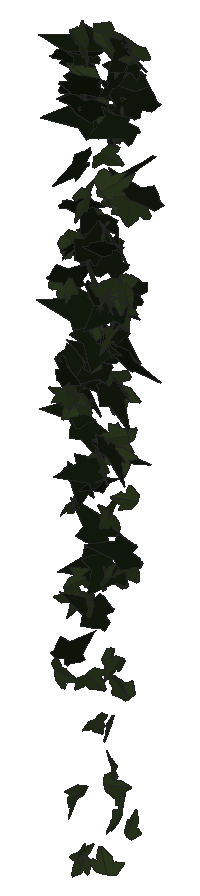
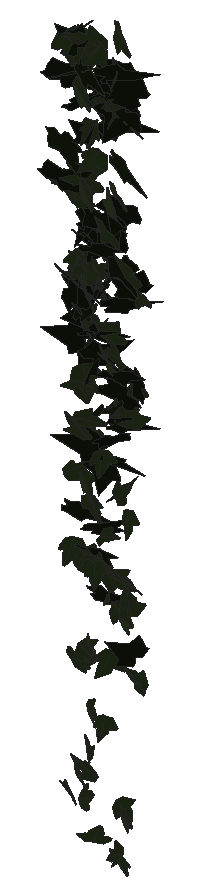
# SketchUp Ruby script. Lengths in inches.
U = 1.inch
M = Sketchup.active_model
def pt(a) = Geom::Point3d.new(a.map { |v| v * U })
def face(e, loops, mat)
  f = e.add_face(loops[0].map { |a| pt(a) })
  loops[1..].each { |l| e.add_face(l.map { |a| pt(a) }).erase! }
  f.material = f.back_material = mat if mat
  f
end
# faces: each face lists its corners as indices into pts; further lists are holes
def faces(e, pts, list, mat = nil) = list.each { |f| face(e, (f[0].is_a?(Array) ? f : [f]).map { |l| l.map { |i| pts[i] } }, mat) }
# xy, xz, yz: faces in a plane at the given z, y or x. An outline is a flat list of corners, or four numbers for a rectangle; further outlines are holes
def ring(l) = l.size == 4 ? [[l[0], l[1]], [l[2], l[1]], [l[2], l[3]], [l[0], l[3]]] : l.each_slice(2).to_a
def flat(e, list, mat, &to3) = list.each { |f| face(e, (f[0].is_a?(Array) ? f : [f]).map { |l| ring(l).map { |u, v| to3.(u, v) } }, mat) }
def xy(e, z, list, mat = nil) = flat(e, list, mat) { |x, y| [x, y, z] }
def xz(e, y, list, mat = nil) = flat(e, list, mat) { |x, z| [x, y, z] }
def yz(e, x, list, mat = nil) = flat(e, list, mat) { |y, z| [x, y, z] }
def lines(e, pts, list) = list.each { |a, b| e.add_line(pt(pts[a]), pt(pts[b])) }
# prism: a flat outline (further loops are holes) pulled along v
def prism(e, loops, v, mat = nil)
  f = face(e, loops, mat); d = Geom::Vector3d.new(v.map { |x| x * U })
  f.pushpull(f.normal.samedirection?(d) ? d.length : -d.length)
end
def box(e, o, s, mat = nil) = prism(e, [[o, [o[0] + s[0], o[1], o[2]], [o[0] + s[0], o[1] + s[1], o[2]], [o[0], o[1] + s[1], o[2]]]], [0, 0, s[2]], mat)
def at(x, y, z, deg = 0) = Geom::Transformation.translation(pt([x, y, z])) * Geom::Transformation.rotation(ORIGIN, Z_AXIS, deg.degrees)
def axes(o, x, y, z) = Geom::Transformation.new([*x, 0, *y, 0, *z, 0, *pt(o).to_a, 1])
def part(name) = M.definitions.add(name)
# library, detail: a bought-in or finely detailed component or shape, given as its bounding box
def library(name, o, s) = part(name).tap { |d| box(d.entities, o, s) }
def detail(e, o, s) = box(e.add_group.entities, o, s)
def put(e, d, t, mat = nil) = e.add_instance(d, t).tap { |i| i.material = mat if mat }
def group(e, t, mat = nil) = e.add_group.tap { |g| g.transformation = t; g.material = mat if mat }.entities
root = M.entities
M.materials.add("1026 AP 7946 SUNNY SIDE UP").color = [254, 231, 186]
M.materials.add("efeu1").color = [18, 25, 13]
M.materials.add("efeu2").color = [43, 57, 29]
c1 = part("ivyleaf_9")
p = [[1.54,2.16,1.25],[1.36,2.04,1.19],[-0.21,0.99,0.68],[-0.71,1.11,0.82],[-0.85,0.86,0.67],[-0.8,0.17,0.21],
  [-0.9,-0.01,0.1],[-0.67,-0.16,-0.02],[-0.08,-0.08,-0.05],[-0.03,-0.6,-0.4],[0.65,-0.88,-0.66],[0.83,-0.6,-0.49],
  [1.29,-0.42,-0.43],[1.8125,-0.07,-0.26],[1.21,0.44,0.15]]
faces(c1.entities,p,[[0,1,2,3,4,5,6,7,8,9,10,11,12,13,14]],"efeu1")
c2 = part("ivyleaf_10")
p = [[0,0.5,-0.03],[-0.0625,2.02,-0.43],[-0.19,2.01,-0.46],[-0.54,1.05,-0.29],[-0.52,0.625,-0.18],[-0.83,0.76,-0.28],
  [-1.16,0.64,-0.33],[-1.15,0.33,-0.24],[-0.77,-0.39,0.02],[-0.3,-0.51,0.16],[0.04,-0.48,0.23],[-0.02,2.01,-0.4375],
  [-0.06,2.01,-0.43],[0.04,-0.49,0.23],[0.67,-0.49,0.14],[1.38,0.36,-0.2],[1.375,0.51,-0.24],[0.81,0.65,-0.19],
  [0.62,0.59,-0.15],[0.6,1.09,-0.28],[0.5,1.23,-0.31]]
faces(c2.entities,p,[[0,1,2,3,4,5,6,7,8,9,10],[11,12,0,13,14,15,16,17,18,19,20]],"efeu2")
put(root,c1,axes([99.77,211.71,258.34],[0.11421,-0.24829,0.05884],[0.0227,-0.05675,-0.26683],[0.40047,0.07403,-0.00166]),"1026 AP 7946 SUNNY SIDE UP")
put(root,c1,axes([100.13,211.37,266.9],[0.01347,0.18196,0.23209],[-0.01628,0.21455,-0.19155],[-0.4771,-0.00219,0.01309]),"1026 AP 7946 SUNNY SIDE UP")
put(root,c1,axes([99.22,211.72,261.21],[-0.20633,0.02031,0.24724],[-0.36489,-0.10681,-0.11268],[0.14623,-0.23786,0.0677]),"1026 AP 7946 SUNNY SIDE UP")
put(root,c2,axes([98.75,211.59,259.34],[-0.065,-0.22355,-0.07009],[0.09307,0.0529,-0.23757],[0.38291,-0.0508,0.04585]),"1026 AP 7946 SUNNY SIDE UP")
put(root,c2,axes([99.16,211.6875,263.875],[0.2789,-0.19863,0.04906],[0.03014,-0.04802,-0.27606],[0.34574,0.16441,-0.01551]),"1026 AP 7946 SUNNY SIDE UP")
put(root,c2,axes([98.63,211.68,261.73],[0.34742,-0.07327,0.07071],[0.09567,-0.04065,-0.23245],[0.13876,0.21148,-0.01677]),"1026 AP 7946 SUNNY SIDE UP")
put(root,c1,axes([98.97,211.53,266.52],[0.37924,0.04384,0.16248],[0.25973,0.0013,-0.24242],[-0.06289,0.26976,-0.02137]),"1026 AP 7946 SUNNY SIDE UP")
put(root,c1,axes([100.32,211.7,256.1],[-0.11456,-0.07824,-0.20637],[-0.2718,-0.10819,0.10608],[-0.22297,0.17209,-0.02328]),"1026 AP 7946 SUNNY SIDE UP")
put(root,c2,axes([99.25,211.52,267.53],[-0.03367,0.04237,0.29564],[-0.39103,0.15321,-0.04082],[-0.26673,-0.22995,0.02253]),"1026 AP 7946 SUNNY SIDE UP")
put(root,c1,axes([99.125,211.71,264.66],[-0.32423,0.16869,-0.09489],[0.08807,-0.07794,-0.27385],[-0.28986,-0.21238,0.02294]),"1026 AP 7946 SUNNY SIDE UP")
put(root,c1,axes([99.38,211.76,257.61],[-0.32792,0.00418,0.0938],[-0.14856,-0.02146,-0.2059],[0.00862,-0.211,0.01982]),"1026 AP 7946 SUNNY SIDE UP")
put(root,c1,axes([99.86,211.79,261.62],[-0.42831,0.01177,-0.06642],[0.10133,-0.04083,-0.26808],[-0.03576,-0.25664,0.03592]),"1026 AP 7946 SUNNY SIDE UP")
put(root,c2,axes([99.64,211.7,261.84],[0.19511,-0.23098,-0.06612],[-0.05478,0.04954,-0.27543],[0.40086,0.1192,-0.00546]),"1026 AP 7946 SUNNY SIDE UP")
put(root,c1,axes([99.79,211.74,259.66],[0.10997,-0.2454,-0.0855],[-0.05012,0.07571,-0.26226],[0.40355,0.07628,-0.00927]),"1026 AP 7946 SUNNY SIDE UP")
put(root,c1,axes([100.0625,211.9,265.8],[-0.25059,-0.12748,0.18092],[-0.19412,-0.12774,-0.20985],[0.30507,-0.186,0.01508]),"1026 AP 7946 SUNNY SIDE UP")
put(root,c1,axes([98.43,211.8125,259.61],[0.17456,-0.11982,-0.18823],[0.345,0.00242,0.12665],[-0.09925,-0.20232,0.10918]),"1026 AP 7946 SUNNY SIDE UP")
put(root,c2,axes([99.34,211.62,262.38],[-0.24271,0.20597,0.10136],[-0.10582,0.0686,-0.2672],[-0.36803,-0.15556,0.00998]),"1026 AP 7946 SUNNY SIDE UP")
put(root,c1,axes([100.12,211.94,267.34],[-0.15431,-0.13846,0.2225],[-0.09689,-0.20573,-0.17483],[0.41533,-0.09944,0.04189]),"1026 AP 7946 SUNNY SIDE UP")
put(root,c2,axes([99.52,211.73,257.96],[-0.22827,0.18235,-0.06401],[0.03856,-0.06028,-0.24273],[-0.32477,-0.13533,0.01617]),"1026 AP 7946 SUNNY SIDE UP")
put(root,c1,axes([99.35,211.61,262.63],[-0.1499,-0.10114,0.24471],[0.27681,0.16226,0.14574],[-0.32428,0.18526,0.01129]),"1026 AP 7946 SUNNY SIDE UP")
put(root,c1,axes([99.39,211.58,262.86],[0.3039,0.19276,0.03365],[0.05358,0.01008,-0.28096],[-0.32651,0.18106,-0.01478]),"1026 AP 7946 SUNNY SIDE UP")
put(root,c2,axes([100.1875,211.84,267.28],[-0.08385,-0.22778,0.11653],[0.005,-0.11442,-0.24974],[0.43071,-0.04302,0.02559]),"1026 AP 7946 SUNNY SIDE UP")
put(root,c1,axes([99.19,211.68,266.08],[0.32051,0.12859,-0.14839],[-0.17988,-0.0931,-0.24535],[-0.26834,0.21601,-0.01277]),"1026 AP 7946 SUNNY SIDE UP")
put(root,c2,axes([99.29,211.67,252.9],[-0.16828,-0.16709,-0.1533],[0.13921,0.11873,-0.20354],[0.32203,-0.13864,0.00787]),"1026 AP 7946 SUNNY SIDE UP")
put(root,c2,axes([98.36,211.82,252.61],[-0.0983,0.03746,0.22474],[0.33412,-0.05251,0.07178],[0.09625,0.22056,-0.01968]),"1026 AP 7946 SUNNY SIDE UP")
put(root,c1,axes([98.63,211.68,261.77],[-0.03622,-0.04414,0.23863],[0.36392,0.07199,0.03814],[-0.13072,0.21263,0.04007]),"1026 AP 7946 SUNNY SIDE UP")
put(root,c2,axes([99.74,211.93,260.85],[0.03742,-0.16086,0.19473],[0.04663,-0.18193,-0.17635],[0.41223,0.03518,0.00227]),"1026 AP 7946 SUNNY SIDE UP")
put(root,c2,axes([99.85,211.84,262],[0.34797,-0.05261,0.13038],[0.19153,-0.05115,-0.2264],[0.12048,0.23324,-0.01666]),"1026 AP 7946 SUNNY SIDE UP")
put(root,c2,axes([99.74,211.77,261.83],[-0.28133,-0.16316,0.06208],[0.05116,0.05488,0.24908],[-0.26918,0.18096,-0.01754]),"1026 AP 7946 SUNNY SIDE UP")
put(root,c1,axes([99.54,211.8,254.375],[-0.24628,-0.09398,-0.16308],[-0.22319,-0.0696,0.18748],[-0.18319,0.21113,-0.00917]),"1026 AP 7946 SUNNY SIDE UP")
put(root,c2,axes([99.83,211.79,261.64],[-0.41731,0.03049,-0.08758],[0.12806,-0.05111,-0.26255],[-0.07583,-0.25412,0.03855]),"1026 AP 7946 SUNNY SIDE UP")
put(root,c1,axes([99.74,211.73,263.22],[0.3409,-0.08165,-0.15278],[-0.22589,0.04871,-0.23136],[0.16125,0.24087,-0.00112]),"1026 AP 7946 SUNNY SIDE UP")
put(root,c1,axes([99.16,211.98,265.65],[-0.06601,-0.11605,-0.26027],[-0.12972,-0.2381,0.12574],[-0.41648,0.09256,0.00209]),"1026 AP 7946 SUNNY SIDE UP")
put(root,c1,axes([99.39,211.96,260.625],[-0.26858,-0.19279,-0.01191],[0.06955,-0.02268,-0.26273],[0.32013,-0.15682,0.04709]),"1026 AP 7946 SUNNY SIDE UP")
put(root,c1,axes([100.39,211.9,266.26],[0.07581,0.0398,0.27726],[-0.43327,-0.05047,0.05483],[0.09667,-0.25739,0.02831]),"1026 AP 7946 SUNNY SIDE UP")
put(root,c1,axes([99.45,211.88,260.0625],[-0.39129,0.04731,-0.05286],[0.0733,-0.03669,-0.25081],[-0.091,-0.23299,0.02529]),"1026 AP 7946 SUNNY SIDE UP")
put(root,c2,axes([99.22,211.89,254.39],[-0.12233,0.18567,0.13228],[0.09489,-0.11261,0.20646],[0.34106,0.09792,-0.01]),"1026 AP 7946 SUNNY SIDE UP")
put(root,c1,axes([99.75,211.6875,262.41],[-0.34926,0.14547,0.01992],[0.04084,0.00516,0.26914],[0.24518,0.20636,-0.01645]),"1026 AP 7946 SUNNY SIDE UP")
put(root,c1,axes([99.43,211.7,257.375],[0.12713,0.19847,0.0268],[0.02228,0.01903,-0.22676],[-0.33832,0.07583,-0.00486]),"1026 AP 7946 SUNNY SIDE UP")
put(root,c1,axes([98.92,211.73,263.65],[0.24636,0.16085,-0.02269],[-0.00791,-0.02709,-0.23178],[-0.27578,0.14447,-0.01362]),"1026 AP 7946 SUNNY SIDE UP")
put(root,c2,axes([99.63,211.79,248.55],[0.25189,0.12326,0.02247],[-0.04422,0.00208,0.20735],[0.1916,-0.16157,0.01831]),"1026 AP 7946 SUNNY SIDE UP")
put(root,c2,axes([99.04,211.94,254.99],[-0.12494,-0.09685,0.18318],[-0.14224,-0.15456,-0.12888],[0.28568,-0.11932,0.01594]),"1026 AP 7946 SUNNY SIDE UP")
put(root,c2,axes([100.11,211.75,262.16],[-0.02207,0.25905,0.06742],[-0.04394,0.05815,-0.27584],[-0.44909,-0.01842,0.02367]),"1026 AP 7946 SUNNY SIDE UP")
put(root,c1,axes([99.65,211.95,255.4375],[-0.34728,-0.09961,-0.02051],[0.04243,-0.013,-0.24856],[0.1538,-0.22132,0.02227]),"1026 AP 7946 SUNNY SIDE UP")
put(root,c1,axes([99.26,211.85,261.77],[0.22541,-0.19793,-0.07928],[-0.0854,0.0522,-0.25411],[0.34687,0.14147,-0.01104]),"1026 AP 7946 SUNNY SIDE UP")
put(root,c1,axes([98.67,211.69,253.14],[-0.0515,-0.01577,0.25538],[0.3206,0.14127,0.03782],[-0.22334,0.20643,-0.00459]),"1026 AP 7946 SUNNY SIDE UP")
put(root,c2,axes([99.77,211.99,266.36],[-0.07588,0.07804,-0.24106],[0.12927,-0.21349,-0.09795],[-0.38505,-0.08705,0.01462]),"1026 AP 7946 SUNNY SIDE UP")
put(root,c2,axes([99.64,211.81,261.62],[-0.21057,0.22314,0.01514],[-0.03009,0.00298,-0.27286],[-0.37807,-0.12452,0.01328]),"1026 AP 7946 SUNNY SIDE UP")
put(root,c1,axes([98.75,212.04,257.13],[-0.02487,-0.2191,0.1306],[0.00606,-0.12846,-0.22676],[0.39897,-0.01171,0.01159]),"1026 AP 7946 SUNNY SIDE UP")
put(root,c2,axes([100.125,211.98,257.11],[0.01722,0.07495,0.19357],[-0.0502,-0.1774,0.07846],[0.32689,-0.03119,0.00185]),"1026 AP 7946 SUNNY SIDE UP")
put(root,c2,axes([100.2,211.87,263.98],[-0.40818,-0.04919,0.04791],[-0.06751,-0.03116,-0.26212],[0.0914,-0.24271,0.02035]),"1026 AP 7946 SUNNY SIDE UP")
put(root,c2,axes([99.86,211.85,258.14],[0.20478,0.16132,0.03611],[0.04892,0.01787,-0.21501],[-0.27474,0.12342,-0.01137]),"1026 AP 7946 SUNNY SIDE UP")
put(root,c2,axes([99.99,211.78,252.81],[-0.0923,0.04532,-0.19893],[-0.2138,0.13771,0.0771],[0.24563,0.13689,-0.00765]),"1026 AP 7946 SUNNY SIDE UP")
put(root,c2,axes([98.63,211.92,254.36],[-0.19793,-0.17291,-0.0116],[-0.0163,-0.00516,0.22023],[-0.27187,0.12619,-0.00476]),"1026 AP 7946 SUNNY SIDE UP")
put(root,c2,axes([99.83,212.01,258.47],[-0.05271,-0.02994,0.20973],[-0.15525,-0.17419,-0.04637],[0.29918,-0.09566,0.01289]),"1026 AP 7946 SUNNY SIDE UP")
put(root,c2,axes([98.94,211.91,248.4375],[0.26207,-0.11136,-0.03687],[-0.06128,0.00472,-0.20569],[0.17309,0.17027,-0.017]),"1026 AP 7946 SUNNY SIDE UP")
put(root,c2,axes([98.79,211.81,259.2],[-0.10666,-0.18282,-0.14148],[0.07852,0.12684,-0.20013],[0.34987,-0.0842,0.00178]),"1026 AP 7946 SUNNY SIDE UP")
put(root,c2,axes([99.78,211.93,257.04],[0.04847,-0.22989,-0.00035],[-0.00813,-0.00167,-0.23889],[0.36139,0.0308,-0.00532]),"1026 AP 7946 SUNNY SIDE UP")
put(root,c1,axes([99.45,212,260.06],[0.01074,0.02465,0.26006],[-0.39443,-0.073,0.01341],[0.12555,-0.23143,0.01988]),"1026 AP 7946 SUNNY SIDE UP")
put(root,c2,axes([99.7,212.07,249.6],[0.03004,-0.04375,0.21059],[0.0993,-0.19474,-0.05009],[0.31375,0.06582,-0.00431]),"1026 AP 7946 SUNNY SIDE UP")
put(root,c2,axes([98.74,211.97,258.9],[0.21961,0.10847,-0.11325],[-0.12403,-0.0793,-0.18141],[-0.22723,0.14812,-0.01043]),"1026 AP 7946 SUNNY SIDE UP")
put(root,c1,axes([99.97,211.92,261.06],[-0.32901,0.15507,-0.0406],[0.03218,-0.04006,-0.2655],[-0.26993,-0.19379,0.01783]),"1026 AP 7946 SUNNY SIDE UP")
put(root,c2,axes([99.67,211.78,255.28],[-0.04216,-0.08694,-0.21107],[0.11142,0.18478,-0.09406],[0.34655,-0.06998,0.00456]),"1026 AP 7946 SUNNY SIDE UP")
put(root,c2,axes([99.51,211.83,255.15],[0.00193,0.02154,0.22739],[-0.32866,0.07351,-0.00577],[-0.11596,-0.20799,0.02013]),"1026 AP 7946 SUNNY SIDE UP")
put(root,c1,axes([99.7,211.96,260.85],[-0.01349,-0.03027,-0.22332],[0.3473,0.04748,-0.01509],[0.08329,-0.20287,0.02675]),"1026 AP 7946 SUNNY SIDE UP")
put(root,c2,axes([99.27,211.89,260.6],[0.3849,0.0616,0.10197],[-0.16573,0.00112,0.25016],[0.09578,-0.24562,0.02307]),"1026 AP 7946 SUNNY SIDE UP")
put(root,c1,axes([99.82,211.98,260.35],[0.26554,-0.0958,0.16998],[0.2094,-0.10351,-0.19688],[0.23747,0.1984,-0.01647]),"1026 AP 7946 SUNNY SIDE UP")
put(root,c1,axes([98.87,212.05,258.68],[-0.22978,-0.02617,0.18399],[-0.27123,-0.06818,-0.1465],[0.11774,-0.20815,0.02159]),"1026 AP 7946 SUNNY SIDE UP")
put(root,c2,axes([98.91,211.92,258.9],[-0.07279,0.01069,0.20005],[-0.31695,-0.01358,-0.04526],[0.01844,-0.1911,0.01172]),"1026 AP 7946 SUNNY SIDE UP")
put(root,c1,axes([99.3,211.9375,263.4],[0.19565,0.07349,-0.18915],[-0.21669,-0.1256,-0.14605],[-0.244,0.17047,-0.02196]),"1026 AP 7946 SUNNY SIDE UP")
put(root,c2,axes([99.66,211.79,264.23],[0.18961,0.06922,-0.23264],[0.2596,0.15811,0.13971],[0.28918,-0.18732,0.02712]),"1026 AP 7946 SUNNY SIDE UP")
put(root,c2,axes([99.15,211.91,259.93],[0.2602,-0.18758,0.04419],[-0.01103,0.05081,0.25847],[-0.32677,-0.15108,0.02647]),"1026 AP 7946 SUNNY SIDE UP")
put(root,c2,axes([99.625,211.93,256.58],[-0.2673,0.07196,0.10474],[-0.17982,-0.00604,-0.17956],[-0.09822,-0.18479,0.04368]),"1026 AP 7946 SUNNY SIDE UP")
put(root,c2,axes([100.06,211.91,252.68],[0.1587,0.00709,0.18049],[-0.28498,0.02229,0.09902],[-0.02731,-0.1914,0.01551]),"1026 AP 7946 SUNNY SIDE UP")
put(root,c1,axes([99.51,212.11,259.7],[0.28166,-0.09472,-0.15865],[0.23244,-0.04677,0.20723],[-0.16242,-0.23119,0.02145]),"1026 AP 7946 SUNNY SIDE UP")
put(root,c1,axes([99.78,212.04,266.8125],[-0.22692,0.14088,-0.15876],[0.14859,-0.12313,-0.20885],[-0.31633,-0.1589,0.01579]),"1026 AP 7946 SUNNY SIDE UP")
put(root,c1,axes([98.83,212.08,259.92],[-0.23827,-0.18294,-0.0634],[0.07847,0.03708,-0.24406],[0.29264,-0.15889,0.01382]),"1026 AP 7946 SUNNY SIDE UP")
put(root,c2,axes([99.52,212.08,251.79],[0.10925,-0.16539,0.10588],[0.0706,-0.0936,-0.1853],[0.29874,0.08261,0.00507]),"1026 AP 7946 SUNNY SIDE UP")
put(root,c2,axes([99.8,212.11,250.17],[0.16008,-0.09453,0.16884],[0.15748,-0.13169,-0.14264],[0.25326,0.14163,-0.01802]),"1026 AP 7946 SUNNY SIDE UP")
put(root,c2,axes([98.63,211.93,256.57],[-0.01894,-0.19773,-0.11195],[0.00578,0.10751,-0.20343],[0.35388,-0.01234,-0.00267]),"1026 AP 7946 SUNNY SIDE UP")
put(root,c2,axes([99.68,212.1,253.18],[-0.05204,-0.17339,0.12318],[0.00106,-0.12212,-0.18146],[0.33206,-0.02679,0.01989]),"1026 AP 7946 SUNNY SIDE UP")
put(root,c1,axes([99.61,212.07,261.47],[0.20511,-0.03374,-0.18171],[0.29137,0.00151,0.13085],[-0.03115,-0.20798,0.02745]),"1026 AP 7946 SUNNY SIDE UP")
put(root,c2,axes([98.79,212.08,254.39],[-0.06672,-0.1879,0.10018],[-0.01489,-0.09849,-0.19869],[0.33312,-0.04203,0.01119]),"1026 AP 7946 SUNNY SIDE UP")
put(root,c2,axes([100.1,211.97,249.49],[0.25581,-0.1377,0.03709],[-0.02408,0.03861,0.2189],[-0.22282,-0.16226,0.01892]),"1026 AP 7946 SUNNY SIDE UP")
put(root,c1,axes([99.83,212.14,267.31],[0.09015,-0.12988,0.20863],[0.15352,-0.17483,-0.15227],[0.36931,0.10438,0.01237]),"1026 AP 7946 SUNNY SIDE UP")
put(root,c1,axes([99.23,212.01,255.3125],[-0.34039,0.13458,0.04242],[-0.07615,-0.00178,-0.26116],[-0.20742,-0.22021,0.02626]),"1026 AP 7946 SUNNY SIDE UP")
put(root,c1,axes([98.93,212.05,258.37],[-0.02421,-0.19811,-0.09633],[0.03472,0.08596,-0.21099],[0.36593,-0.02127,0.01365]),"1026 AP 7946 SUNNY SIDE UP")
put(root,c2,axes([98.59,212.04,258.89],[-0.39452,-0.06468,0.02264],[0.03434,0.00479,0.26695],[-0.10198,0.25185,0.00231]),"1026 AP 7946 SUNNY SIDE UP")
put(root,c2,axes([99.33,211.97,266.01],[0.2022,-0.11148,-0.22863],[-0.30782,0.10714,-0.17217],[0.23886,0.23244,-0.02834]),"1026 AP 7946 SUNNY SIDE UP")
put(root,c2,axes([99.68,212.18,263.79],[-0.0596,0.06232,0.24131],[0.03144,-0.22566,0.06699],[0.3944,0.02741,0.03112]),"1026 AP 7946 SUNNY SIDE UP")
put(root,c2,axes([98.85,212.17,266.02],[0.00901,0.10107,-0.22834],[-0.01675,-0.21438,-0.11134],[-0.40233,0.01119,-0.00048]),"1026 AP 7946 SUNNY SIDE UP")
put(root,c2,axes([99.07,212.11,263.1875],[0.32623,-0.06448,0.17185],[0.23628,-0.07671,-0.22304],[0.15347,0.25516,-0.0219]),"1026 AP 7946 SUNNY SIDE UP")
put(root,c2,axes([98.99,211.93,266.05],[-0.19672,0.16519,0.11118],[-0.12548,0.07192,-0.21424],[-0.30445,-0.13638,0.01646]),"1026 AP 7946 SUNNY SIDE UP")
put(root,c2,axes([99.47,212.12,253.29],[0.2006,-0.12606,0.11295],[0.09984,-0.09198,-0.1844],[0.24379,0.1414,-0.01742]),"1026 AP 7946 SUNNY SIDE UP")
put(root,c2,axes([99.69,212.08,261.71],[0.17031,-0.23035,0.01981],[-0.00094,-0.02295,-0.26215],[0.36364,0.10783,-0.00996]),"1026 AP 7946 SUNNY SIDE UP")
put(root,c2,axes([99.69,212.05,264.11],[0.36968,0.09927,0.03132],[0.0578,-0.00753,-0.25536],[-0.16526,0.21943,-0.01925]),"1026 AP 7946 SUNNY SIDE UP")
put(root,c2,axes([98.5625,212.17,254.26],[0.10403,-0.13645,0.16431],[0.08717,-0.15078,-0.1567],[0.31929,0.08562,-0.01076]),"1026 AP 7946 SUNNY SIDE UP")
put(root,c1,axes([99.09,212.02,266.05],[-0.29294,0.13389,0.05109],[-0.08498,0.01008,-0.23247],[-0.22478,-0.1783,0.02131]),"1026 AP 7946 SUNNY SIDE UP")
put(root,c1,axes([99.4,212.06,256.04],[-0.30277,-0.17476,-0.01068],[-0.03059,0.00752,0.26724],[-0.27348,0.19263,-0.01807]),"1026 AP 7946 SUNNY SIDE UP")
put(root,c1,axes([100.37,211.9375,264.88],[-0.09154,0.26283,0.01344],[-0.03386,0.00521,-0.28649],[-0.44515,-0.05444,0.01902]),"1026 AP 7946 SUNNY SIDE UP")
put(root,c2,axes([99.25,212.05,257.8125],[-0.12666,-0.19298,-0.03668],[0.05728,0.02077,-0.21976],[0.32702,-0.07838,0.02429]),"1026 AP 7946 SUNNY SIDE UP")
put(root,c2,axes([98.86,212.18,263.75],[0.01694,-0.16192,-0.17114],[0.08821,-0.15203,0.16846],[-0.37346,-0.04325,0.03203]),"1026 AP 7946 SUNNY SIDE UP")
put(root,c2,axes([99.1,212.16,256.05],[0.08269,0.06532,-0.16749],[-0.13375,-0.13641,-0.08867],[-0.25634,0.09224,-0.00776]),"1026 AP 7946 SUNNY SIDE UP")
put(root,c1,axes([99.98,212.17,261.54],[-0.10142,0.07217,-0.22361],[0.18254,-0.18064,-0.10183],[-0.32946,-0.12231,0.01242]),"1026 AP 7946 SUNNY SIDE UP")
put(root,c2,axes([99.47,212.11,250.29],[0.10265,-0.05641,-0.20523],[0.27358,-0.09766,0.08679],[-0.17557,-0.18516,0.01526]),"1026 AP 7946 SUNNY SIDE UP")
put(root,c2,axes([99.49,212.13,250.7],[-0.14478,0.09118,0.17164],[0.2132,-0.09727,0.13188],[0.2081,0.1631,-0.01571]),"1026 AP 7946 SUNNY SIDE UP")
put(root,c1,axes([99.35,212.2,262.77],[-0.33338,-0.12675,0.01829],[-0.00812,-0.02724,-0.25375],[0.20125,-0.21107,0.02006]),"1026 AP 7946 SUNNY SIDE UP")
put(root,c2,axes([98.89,211.92,248.5],[0.02531,-0.05452,0.2005],[-0.07945,0.18828,0.05965],[-0.3082,-0.05301,0.00109]),"1026 AP 7946 SUNNY SIDE UP")
put(root,c1,axes([98.68,212.11,259.33],[0.20638,-0.20228,-0.02344],[-0.02938,0.01361,-0.24819],[0.31852,0.13232,-0.0077]),"1026 AP 7946 SUNNY SIDE UP")
put(root,c1,axes([99.375,212.04,257.93],[0.19573,-0.00725,0.21311],[0.31583,-0.05432,-0.12676],[0.07895,0.23528,-0.02125]),"1026 AP 7946 SUNNY SIDE UP")
put(root,c2,axes([98.53,212.18,249.61],[0.09745,-0.15235,0.12079],[0.07513,-0.10805,-0.17005],[0.29366,0.07821,0.00342]),"1026 AP 7946 SUNNY SIDE UP")
put(root,c1,axes([98.73,212.04,262.54],[-0.05449,0.20761,-0.08748],[0.0273,-0.08293,-0.22604],[-0.37947,-0.03578,-0.0037]),"1026 AP 7946 SUNNY SIDE UP")
put(root,c2,axes([98.66,212.16,249.86],[-0.0566,-0.18504,0.08677],[-0.01888,-0.08452,-0.19465],[0.31981,-0.03774,0.00386]),"1026 AP 7946 SUNNY SIDE UP")
put(root,c2,axes([98.625,212.25,257.18],[-0.0402,-0.06148,-0.21105],[-0.09016,-0.19644,0.06707],[-0.32347,0.0624,0.00753]),"1026 AP 7946 SUNNY SIDE UP")
put(root,c2,axes([99.84,212.03,255.12],[-0.19453,0.0752,-0.15874],[-0.20018,0.09186,0.14776],[0.20104,0.16423,-0.00647]),"1026 AP 7946 SUNNY SIDE UP")
put(root,c2,axes([100.01,212.1,267.375],[-0.34632,-0.15472,0.01984],[-0.00512,-0.0299,-0.27353],[0.2649,-0.20285,0.02064]),"1026 AP 7946 SUNNY SIDE UP")
put(root,c2,axes([98.76,212.22,267.09],[-0.06837,0.126,-0.21183],[0.07667,-0.19454,-0.14401],[-0.39316,-0.05984,0.00875]),"1026 AP 7946 SUNNY SIDE UP")
put(root,c1,axes([99.52,212.1,260.46],[-0.0418,-0.20079,0.12083],[0.03856,0.11348,0.218],[-0.3913,0.03263,0.00858]),"1026 AP 7946 SUNNY SIDE UP")
put(root,c1,axes([98.56,212.11,259.54],[0.06537,-0.07691,-0.23332],[0.32738,0.124,-0.00329],[0.18379,-0.19351,0.08885]),"1026 AP 7946 SUNNY SIDE UP")
put(root,c2,axes([99.5,212.0625,265.49],[-0.29597,0.13713,0.02338],[-0.04691,-0.00283,-0.23662],[-0.23054,-0.17548,0.01813]),"1026 AP 7946 SUNNY SIDE UP")
put(root,c1,axes([98.35,212.06,266.61],[0.3236,0.1456,-0.06451],[0.06004,0.05565,0.2565],[0.26195,-0.19263,0.0209]),"1026 AP 7946 SUNNY SIDE UP")
put(root,c2,axes([99.41,212.01,264.8125],[-0.14235,-0.13264,-0.17346],[0.16676,0.1271,-0.16585],[0.31134,-0.12873,0.00952]),"1026 AP 7946 SUNNY SIDE UP")
put(root,c2,axes([99.49,212.17,261.99],[-0.28269,0.16365,0.12246],[0.14496,-0.07386,0.24993],[0.28212,0.20193,-0.00571]),"1026 AP 7946 SUNNY SIDE UP")
put(root,c2,axes([100,212.0625,255.51],[-0.14461,-0.19364,-0.09465],[0.08771,0.07367,-0.21969],[0.32463,-0.10616,0.01719]),"1026 AP 7946 SUNNY SIDE UP")
put(root,c1,axes([98.9375,212.23,266.9375],[-0.1784,0.01715,0.26165],[-0.39129,-0.06554,-0.11038],[0.08358,-0.27024,0.0417]),"1026 AP 7946 SUNNY SIDE UP")
put(root,c2,axes([99.32,212.13,267.43],[-0.36583,0.11589,-0.11417],[0.13313,-0.0784,-0.26646],[-0.21496,-0.24578,0.02926]),"1026 AP 7946 SUNNY SIDE UP")
put(root,c1,axes([100.34,212.09,263.95],[0.07488,0.02259,0.25862],[-0.36258,0.11947,0.0315],[-0.19432,-0.21421,0.04089]),"1026 AP 7946 SUNNY SIDE UP")
put(root,c2,axes([98.4,212.15,262.4],[0.19825,0.01867,0.24205],[0.37044,-0.00981,-0.12955],[-0.00025,0.26637,-0.02017]),"1026 AP 7946 SUNNY SIDE UP")
put(root,c2,axes([99.38,212.1,255.18],[-0.10088,-0.20699,-0.0466],[0.02195,0.0418,-0.223],[0.33204,-0.06565,0.00058]),"1026 AP 7946 SUNNY SIDE UP")
put(root,c1,axes([99.625,212.22,261.09],[0.14518,-0.20969,0.02872],[0.00774,0.03369,0.24224],[-0.35939,-0.08398,0.01682]),"1026 AP 7946 SUNNY SIDE UP")
put(root,c2,axes([99.71,212.23,266.39],[0.12584,-0.24777,0.08823],[0.02274,-0.0867,-0.26844],[0.41231,0.0804,-0.01212]),"1026 AP 7946 SUNNY SIDE UP")
put(root,c1,axes([100.2,212.09,261.81],[-0.27757,0.14359,0.09473],[-0.13196,0.04229,-0.23157],[-0.25224,-0.18014,0.0169]),"1026 AP 7946 SUNNY SIDE UP")
put(root,c1,axes([99.86,212.32,266.72],[-0.19753,-0.20333,0.08789],[0.05687,-0.11106,-0.23758],[0.36959,-0.09158,0.08353]),"1026 AP 7946 SUNNY SIDE UP")
put(root,c2,axes([99.3,212.09,267.49],[-0.00109,-0.00721,0.26471],[0.39112,0.09023,0.00472],[-0.15326,0.23031,0.01015]),"1026 AP 7946 SUNNY SIDE UP")
put(root,c2,axes([99.64,212.16,259.39],[0.34417,0.10084,-0.0185],[-0.01204,-0.02731,-0.24174],[-0.17366,0.20176,-0.0199]),"1026 AP 7946 SUNNY SIDE UP")
put(root,c2,axes([99.62,212.15,259.74],[-0.20078,-0.20225,0.00288],[0.00779,-0.00886,-0.2508],[0.34337,-0.11807,0.00738]),"1026 AP 7946 SUNNY SIDE UP")
put(root,c2,axes([99.49,212.05,265.53],[-0.02061,0.20622,0.09363],[-0.00812,0.08463,-0.21998],[-0.3784,-0.01305,-0.00038]),"1026 AP 7946 SUNNY SIDE UP")
put(root,c2,axes([98.86,212.21,266.26],[0.0239,0.18318,0.13815],[-0.10108,-0.11919,0.18998],[0.36429,-0.04509,0.04365]),"1026 AP 7946 SUNNY SIDE UP")
put(root,c1,axes([99.46,212.04,265.25],[-0.12209,-0.01858,0.22505],[0.31804,0.09714,0.07908],[-0.16576,0.20007,-0.01402]),"1026 AP 7946 SUNNY SIDE UP")
put(root,c2,axes([99.125,212.1,251.64],[-0.10266,-0.17653,-0.09162],[0.05989,0.07959,-0.19329],[0.30427,-0.07523,0.00713]),"1026 AP 7946 SUNNY SIDE UP")
put(root,c2,axes([98.66,212.24,260.43],[0.12736,-0.02629,0.21542],[0.31616,-0.07718,-0.08607],[0.13822,0.20075,-0.00162]),"1026 AP 7946 SUNNY SIDE UP")
put(root,c2,axes([99.58,212.21,264.08],[0.08242,-0.23244,0.02838],[-0.00236,-0.02991,-0.24551],[0.3683,0.05182,-0.00792]),"1026 AP 7946 SUNNY SIDE UP")
put(root,c2,axes([99.625,212.17,258.26],[0.25335,-0.08645,-0.13307],[0.19976,-0.03273,0.18634],[-0.1397,-0.20359,0.02511]),"1026 AP 7946 SUNNY SIDE UP")
put(root,c1,axes([98.65,212.04,266.09],[0.32208,0.14995,-0.00199],[0.0142,-0.01671,-0.25839],[-0.25423,0.18903,-0.01695]),"1026 AP 7946 SUNNY SIDE UP")
